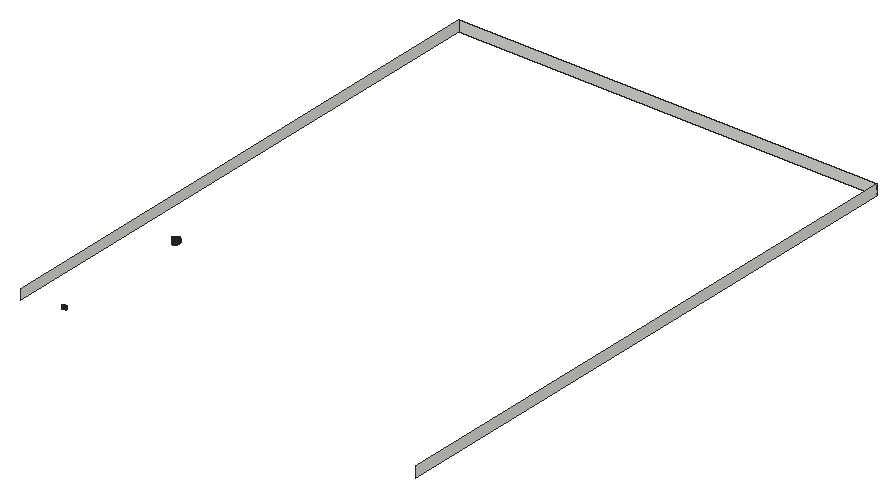
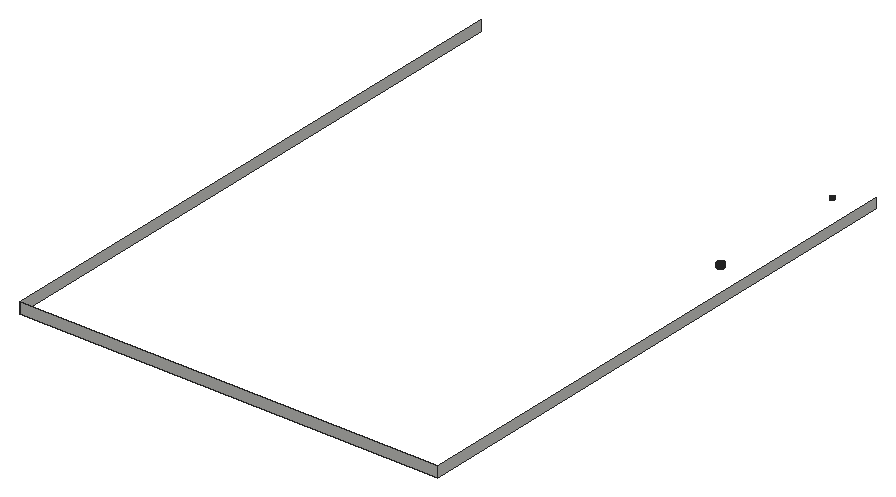
# SketchUp Ruby script. Lengths in inches.
U = 1.inch
M = Sketchup.active_model
def pt(a) = Geom::Point3d.new(a.map { |v| v * U })
def face(e, loops, mat)
  f = e.add_face(loops[0].map { |a| pt(a) })
  loops[1..].each { |l| e.add_face(l.map { |a| pt(a) }).erase! }
  f.material = f.back_material = mat if mat
  f
end
# faces: each face lists its corners as indices into pts; further lists are holes
def faces(e, pts, list, mat = nil) = list.each { |f| face(e, (f[0].is_a?(Array) ? f : [f]).map { |l| l.map { |i| pts[i] } }, mat) }
# xy, xz, yz: faces in a plane at the given z, y or x. An outline is a flat list of corners, or four numbers for a rectangle; further outlines are holes
def ring(l) = l.size == 4 ? [[l[0], l[1]], [l[2], l[1]], [l[2], l[3]], [l[0], l[3]]] : l.each_slice(2).to_a
def flat(e, list, mat, &to3) = list.each { |f| face(e, (f[0].is_a?(Array) ? f : [f]).map { |l| ring(l).map { |u, v| to3.(u, v) } }, mat) }
def xy(e, z, list, mat = nil) = flat(e, list, mat) { |x, y| [x, y, z] }
def xz(e, y, list, mat = nil) = flat(e, list, mat) { |x, z| [x, y, z] }
def yz(e, x, list, mat = nil) = flat(e, list, mat) { |y, z| [x, y, z] }
def lines(e, pts, list) = list.each { |a, b| e.add_line(pt(pts[a]), pt(pts[b])) }
# prism: a flat outline (further loops are holes) pulled along v
def prism(e, loops, v, mat = nil)
  f = face(e, loops, mat); d = Geom::Vector3d.new(v.map { |x| x * U })
  f.pushpull(f.normal.samedirection?(d) ? d.length : -d.length)
end
def box(e, o, s, mat = nil) = prism(e, [[o, [o[0] + s[0], o[1], o[2]], [o[0] + s[0], o[1] + s[1], o[2]], [o[0], o[1] + s[1], o[2]]]], [0, 0, s[2]], mat)
def at(x, y, z, deg = 0) = Geom::Transformation.translation(pt([x, y, z])) * Geom::Transformation.rotation(ORIGIN, Z_AXIS, deg.degrees)
def axes(o, x, y, z) = Geom::Transformation.new([*x, 0, *y, 0, *z, 0, *pt(o).to_a, 1])
def part(name) = M.definitions.add(name)
# library, detail: a bought-in or finely detailed component or shape, given as its bounding box
def library(name, o, s) = part(name).tap { |d| box(d.entities, o, s) }
def detail(e, o, s) = box(e.add_group.entities, o, s)
def put(e, d, t, mat = nil) = e.add_instance(d, t).tap { |i| i.material = mat if mat }
def group(e, t, mat = nil) = e.add_group.tap { |g| g.transformation = t; g.material = mat if mat }.entities
root = M.entities
M.materials.add("1122 AP 7994 PEACH ROSE").color = [254, 227, 201]
xz(root,186.05,[[40.625,149.82,40.7,152.82],[41.33,149.82,41.41,152.82]],"1122 AP 7994 PEACH ROSE")
xz(root,186.07,[[40.86,149.82,40.9375,152.82],[40.9375,149.82,41.02,152.82],[41.02,149.82,41.09,152.82],[41.09,149.82,41.17,152.82]],"1122 AP 7994 PEACH ROSE")
xz(root,300.07,[[40.86,149.82,40.9375,152.82],[40.9375,149.82,41.02,152.82],[41.02,149.82,41.09,152.82],[41.09,149.82,41.17,152.82]],"1122 AP 7994 PEACH ROSE")
xz(root,306.05,[[40.625,149.82,40.7,152.82],[41.33,149.82,41.41,152.82]],"1122 AP 7994 PEACH ROSE")
xz(root,306.07,[[40.86,149.82,40.9375,152.82],[40.9375,149.82,41.02,152.82],[41.02,149.82,41.09,152.82],[41.09,149.82,41.17,152.82]],"1122 AP 7994 PEACH ROSE")
xz(root,645,[[9,149.82,366,158.82]])
yz(root,9,[[177,149.82,645,158.82]])
yz(root,38.02,[[302.91,149.82,302.99,152.82],[302.99,149.82,303.07,152.82],[303.07,149.82,303.15,152.82],[303.15,149.82,303.23,152.82]],"1122 AP 7994 PEACH ROSE")
yz(root,38.03,[[302.76,149.82,302.84,152.82],[303.31,149.82,303.38,152.82]],"1122 AP 7994 PEACH ROSE")
yz(root,44.01,[[302.84,149.82,302.91,152.82],[303.23,149.82,303.31,152.82]],"1122 AP 7994 PEACH ROSE")
yz(root,44.02,[[302.99,149.82,303.07,152.82],[303.07,149.82,303.15,152.82]],"1122 AP 7994 PEACH ROSE")
yz(root,366,[[153,149.82,645,158.82]])
p = [[38.38,184.5,149.82],[38.42,184.57,149.82],[38.42,184.57,152.82],[38.38,184.5,152.82],[38.46,184.64,149.82],[38.46,184.64,152.82],
  [38.5,184.7,149.82],[38.5,184.7,152.82],[38.54,184.77,149.82],[38.54,184.77,152.82],[38.59,184.83,149.82],[38.59,184.83,152.82],
  [38.64,184.9,149.82],[38.64,184.9,152.82],[38.68,184.96,149.82],[38.68,184.96,152.82],[38.74,185.02,149.82],[38.74,185.02,152.82],
  [38.79,185.08,149.82],[38.79,185.08,152.82],[38.84,185.14,149.82],[38.84,185.14,152.82],[38.89,185.19,149.82],[38.89,185.19,152.82],
  [38.95,185.25,149.82],[38.95,185.25,152.82],[39.01,185.3,149.82],[39.01,185.3,152.82],[39.07,185.35,149.82],[39.07,185.35,152.82],
  [39.13,185.4,149.82],[39.13,185.4,152.82],[39.19,185.45,149.82],[39.19,185.45,152.82],[39.25,185.5,149.82],[39.25,185.5,152.82],
  [39.32,185.54,149.82],[39.32,185.54,152.82],[39.38,185.59,149.82],[39.38,185.59,152.82],[39.45,185.63,149.82],[39.45,185.63,152.82],
  [39.52,185.67,149.82],[39.52,185.67,152.82],[39.58,185.71,149.82],[39.58,185.71,152.82],[39.65,185.74,149.82],[39.65,185.74,152.82],
  [39.72,185.78,149.82],[39.72,185.78,152.82],[39.8,185.8125,149.82],[39.8,185.8125,152.82],[39.87,185.84,149.82],[39.87,185.84,152.82],
  [39.94,185.87,149.82],[39.94,185.87,152.82],[40.01,185.9,149.82],[40.01,185.9,152.82],[40.09,185.92,149.82],[40.09,185.92,152.82],
  [40.16,185.95,149.82],[40.16,185.95,152.82],[40.24,185.97,149.82],[40.24,185.97,152.82],[40.32,185.99,149.82],[40.32,185.99,152.82],
  [40.39,186.01,149.82],[40.39,186.01,152.82],[40.47,186.02,149.82],[40.47,186.02,152.82],[40.55,186.03,149.82],[40.55,186.03,152.82],
  [40.625,186.05,149.82],[40.625,186.05,152.82],[41.41,186.05,149.82],[41.49,186.03,149.82],[41.49,186.03,152.82],[41.41,186.05,152.82],
  [41.5625,186.02,149.82],[41.5625,186.02,152.82],[41.64,186.01,149.82],[41.64,186.01,152.82],[40.7,186.05,149.82],[40.78,186.0625,149.82],
  [40.78,186.0625,152.82],[40.7,186.05,152.82],[40.86,186.07,149.82],[40.86,186.07,152.82],[41.17,186.07,149.82],[41.25,186.0625,149.82],
  [41.25,186.0625,152.82],[41.17,186.07,152.82],[41.33,186.05,149.82],[41.33,186.05,152.82],[40.39,300.14,149.82],[40.32,300.15,149.82],
  [40.32,300.15,152.82],[40.39,300.14,152.82],[40.47,300.12,149.82],[40.47,300.12,152.82],[40.625,300.1,149.82],[40.55,300.11,149.82],
  [40.55,300.11,152.82],[40.625,300.1,152.82],[40.7,300.09,149.82],[40.7,300.09,152.82],[40.78,300.08,149.82],[40.78,300.08,152.82],
  [40.86,300.07,149.82],[40.86,300.07,152.82],[41.25,300.08,149.82],[41.17,300.07,149.82],[41.17,300.07,152.82],[41.25,300.08,152.82],
  [41.33,300.09,149.82],[41.33,300.09,152.82],[41.41,300.1,149.82],[41.41,300.1,152.82],[41.49,300.11,149.82],[41.49,300.11,152.82],
  [41.5625,300.12,149.82],[41.5625,300.12,152.82],[41.64,300.14,149.82],[41.64,300.14,152.82],[41.72,300.15,149.82],[41.72,300.15,152.82],
  [40.01,300.24,149.82],[39.94,300.27,149.82],[39.94,300.27,152.82],[40.01,300.24,152.82],[40.09,300.22,149.82],[40.09,300.22,152.82],
  [40.16,300.19,149.82],[40.16,300.19,152.82],[40.24,300.17,149.82],[40.24,300.17,152.82],[41.79,300.17,149.82],[41.79,300.17,152.82],
  [41.87,300.19,149.82],[41.87,300.19,152.82],[41.94,300.22,149.82],[41.94,300.22,152.82],[42.02,300.24,149.82],[42.02,300.24,152.82],
  [42.09,300.27,149.82],[42.09,300.27,152.82],[39.8,300.33,149.82],[39.72,300.36,149.82],[39.72,300.36,152.82],[39.8,300.33,152.82],
  [39.87,300.3,149.82],[39.87,300.3,152.82],[42.16,300.3,149.82],[42.16,300.3,152.82],[42.24,300.33,149.82],[42.24,300.33,152.82],
  [42.31,300.36,149.82],[42.31,300.36,152.82],[39.58,300.43,149.82],[39.52,300.47,149.82],[39.52,300.47,152.82],[39.58,300.43,152.82],
  [39.65,300.4,149.82],[39.65,300.4,152.82],[42.38,300.4,149.82],[42.38,300.4,152.82],[42.45,300.43,149.82],[42.45,300.43,152.82],
  [42.52,300.47,149.82],[42.52,300.47,152.82],[39.45,300.51,149.82],[39.45,300.51,152.82],[39.38,300.55,149.82],[39.38,300.55,152.82],
  [42.58,300.51,149.82],[42.58,300.51,152.82],[42.65,300.55,149.82],[42.65,300.55,152.82],[39.25,300.64,149.82],[39.19,300.69,149.82],
  [39.19,300.69,152.82],[39.25,300.64,152.82],[39.32,300.6,149.82],[39.32,300.6,152.82],[42.72,300.6,149.82],[42.72,300.6,152.82],
  [42.78,300.64,149.82],[42.78,300.64,152.82],[42.84,300.69,149.82],[42.84,300.69,152.82],[39.13,300.74,149.82],[39.13,300.74,152.82],
  [39.07,300.79,149.82],[39.07,300.79,152.82],[42.9,300.74,149.82],[42.9,300.74,152.82],[42.96,300.79,149.82],[42.96,300.79,152.82],
  [39.01,300.84,149.82],[39.01,300.84,152.82],[38.95,300.89,149.82],[38.95,300.89,152.82],[43.02,300.84,149.82],[43.02,300.84,152.82],
  [43.08,300.89,149.82],[43.08,300.89,152.82],[38.89,300.95,149.82],[38.84,301.01,149.82],[38.84,301.01,152.82],[38.89,300.95,152.82],
  [43.14,300.95,149.82],[43.14,300.95,152.82],[43.19,301.01,149.82],[43.19,301.01,152.82],[38.79,301.0625,149.82],[38.79,301.0625,152.82],
  [43.25,301.0625,149.82],[43.25,301.0625,152.82],[38.74,301.12,149.82],[38.74,301.12,152.82],[38.68,301.18,149.82],[38.68,301.18,152.82],
  [43.3,301.12,149.82],[43.3,301.12,152.82],[43.35,301.18,149.82],[43.35,301.18,152.82],[38.64,301.24,149.82],[38.64,301.24,152.82],
  [38.59,301.31,149.82],[38.59,301.31,152.82],[43.4,301.24,149.82],[43.4,301.24,152.82],[43.44,301.31,149.82],[43.44,301.31,152.82],
  [38.54,301.37,149.82],[38.54,301.37,152.82],[43.49,301.37,149.82],[43.49,301.37,152.82],[38.5,301.4375,149.82],[38.5,301.4375,152.82],
  [38.46,301.5,149.82],[38.46,301.5,152.82],[43.53,301.4375,149.82],[43.53,301.4375,152.82],[43.57,301.5,149.82],[43.57,301.5,152.82],
  [38.42,301.57,149.82],[38.42,301.57,152.82],[43.61,301.57,149.82],[43.61,301.57,152.82],[38.38,301.64,149.82],[38.34,301.71,149.82],
  [38.34,301.71,152.82],[38.38,301.64,152.82],[43.65,301.64,149.82],[43.65,301.64,152.82],[43.6875,301.71,149.82],[43.6875,301.71,152.82],
  [38.31,301.78,149.82],[38.31,301.78,152.82],[43.72,301.78,149.82],[43.72,301.78,152.82],[38.28,301.85,149.82],[38.28,301.85,152.82],
  [43.76,301.85,149.82],[43.76,301.85,152.82],[38.24,301.92,149.82],[38.24,301.92,152.82],[38.22,302,149.82],[38.22,302,152.82],
  [43.79,301.92,149.82],[43.79,301.92,152.82],[43.82,302,149.82],[43.82,302,152.82],[38.1875,302.07,149.82],[38.1875,302.07,152.82],
  [43.84,302.07,149.82],[43.84,302.07,152.82],[38.16,302.14,149.82],[38.14,302.22,149.82],[38.14,302.22,152.82],[38.16,302.14,152.82],
  [43.87,302.14,149.82],[43.87,302.14,152.82],[43.89,302.22,149.82],[43.89,302.22,152.82],[38.12,302.29,149.82],[38.12,302.29,152.82],
  [43.91,302.29,149.82],[43.91,302.29,152.82],[38.1,302.37,149.82],[38.1,302.37,152.82],[43.93,302.37,149.82],[43.93,302.37,152.82],
  [38.08,302.45,149.82],[38.08,302.45,152.82],[38.07,302.52,149.82],[38.07,302.52,152.82],[43.95,302.45,149.82],[43.95,302.45,152.82],
  [43.97,302.52,149.82],[43.97,302.52,152.82],[38.05,302.6,149.82],[38.05,302.6,152.82],[43.98,302.6,149.82],[43.98,302.6,152.82],
  [38.04,302.68,149.82],[38.04,302.68,152.82],[43.99,302.68,149.82],[43.99,302.68,152.82],[38.03,302.76,149.82],[38.03,302.76,152.82],
  [44,302.76,149.82],[44,302.76,152.82],[38.03,302.84,149.82],[38.02,302.91,149.82],[38.02,302.91,152.82],[38.03,302.84,152.82],
  [44.01,302.84,149.82],[44.01,302.84,152.82],[44.02,302.99,149.82],[44.01,302.91,149.82],[44.01,302.91,152.82],[44.02,302.99,152.82],
  [44.01,303.23,149.82],[44.02,303.15,149.82],[44.02,303.15,152.82],[44.01,303.23,152.82],[38.02,303.23,149.82],[38.03,303.31,149.82],
  [38.03,303.31,152.82],[38.02,303.23,152.82],[44,303.38,149.82],[44.01,303.31,149.82],[44.01,303.31,152.82],[44,303.38,152.82],
  [38.03,303.38,149.82],[38.04,303.46,149.82],[38.04,303.46,152.82],[38.03,303.38,152.82],[43.99,303.46,149.82],[43.99,303.46,152.82],
  [38.05,303.54,149.82],[38.05,303.54,152.82],[38.07,303.62,149.82],[38.07,303.62,152.82],[43.98,303.54,149.82],[43.98,303.54,152.82],
  [43.97,303.62,149.82],[43.97,303.62,152.82],[38.08,303.69,149.82],[38.08,303.69,152.82],[43.95,303.69,149.82],[43.95,303.69,152.82],
  [38.1,303.77,149.82],[38.1,303.77,152.82],[43.93,303.77,149.82],[43.93,303.77,152.82],[38.12,303.85,149.82],[38.12,303.85,152.82],
  [38.14,303.92,149.82],[38.14,303.92,152.82],[43.91,303.85,149.82],[43.91,303.85,152.82],[43.89,303.92,149.82],[43.89,303.92,152.82],
  [38.16,304,149.82],[38.16,304,152.82],[43.87,304,149.82],[43.87,304,152.82],[38.1875,304.07,149.82],[38.1875,304.07,152.82],
  [43.84,304.07,149.82],[43.84,304.07,152.82],[38.22,304.15,149.82],[38.22,304.15,152.82],[38.24,304.22,149.82],[38.24,304.22,152.82],
  [43.82,304.15,149.82],[43.82,304.15,152.82],[43.79,304.22,149.82],[43.79,304.22,152.82],[38.28,304.29,149.82],[38.28,304.29,152.82],
  [43.76,304.29,149.82],[43.76,304.29,152.82],[38.31,304.36,149.82],[38.31,304.36,152.82],[43.72,304.36,149.82],[43.72,304.36,152.82],
  [38.34,304.43,149.82],[38.34,304.43,152.82],[38.38,304.5,149.82],[38.38,304.5,152.82],[43.6875,304.43,149.82],[43.6875,304.43,152.82],
  [43.65,304.5,149.82],[43.65,304.5,152.82],[38.42,304.57,149.82],[38.42,304.57,152.82],[43.61,304.57,149.82],[43.61,304.57,152.82],
  [38.46,304.64,149.82],[38.46,304.64,152.82],[38.5,304.7,149.82],[38.5,304.7,152.82],[43.53,304.7,149.82],[43.57,304.64,149.82],
  [43.57,304.64,152.82],[43.53,304.7,152.82],[38.54,304.77,149.82],[38.54,304.77,152.82],[43.49,304.77,149.82],[43.49,304.77,152.82],
  [38.59,304.83,149.82],[38.59,304.83,152.82],[38.64,304.9,149.82],[38.64,304.9,152.82],[43.44,304.83,149.82],[43.44,304.83,152.82],
  [43.4,304.9,149.82],[43.4,304.9,152.82],[38.68,304.96,149.82],[38.68,304.96,152.82],[43.35,304.96,149.82],[43.35,304.96,152.82],
  [38.74,305.02,149.82],[38.74,305.02,152.82],[38.79,305.08,149.82],[38.79,305.08,152.82],[43.25,305.08,149.82],[43.3,305.02,149.82],
  [43.3,305.02,152.82],[43.25,305.08,152.82],[38.84,305.14,149.82],[38.84,305.14,152.82],[38.89,305.19,149.82],[38.89,305.19,152.82],
  [43.14,305.19,149.82],[43.19,305.14,149.82],[43.19,305.14,152.82],[43.14,305.19,152.82],[38.95,305.25,149.82],[38.95,305.25,152.82],
  [39.01,305.3,149.82],[39.01,305.3,152.82],[43.02,305.3,149.82],[43.08,305.25,149.82],[43.08,305.25,152.82],[43.02,305.3,152.82],
  [39.07,305.35,149.82],[39.07,305.35,152.82],[42.96,305.35,149.82],[42.96,305.35,152.82],[39.13,305.4,149.82],[39.13,305.4,152.82],
  [39.19,305.45,149.82],[39.19,305.45,152.82],[42.84,305.45,149.82],[42.9,305.4,149.82],[42.9,305.4,152.82],[42.84,305.45,152.82],
  [39.25,305.5,149.82],[39.25,305.5,152.82],[39.32,305.54,149.82],[39.32,305.54,152.82],[39.38,305.59,149.82],[39.38,305.59,152.82],
  [42.72,305.54,149.82],[42.78,305.5,149.82],[42.78,305.5,152.82],[42.72,305.54,152.82],[42.65,305.59,149.82],[42.65,305.59,152.82],
  [39.45,305.63,149.82],[39.45,305.63,152.82],[39.52,305.67,149.82],[39.52,305.67,152.82],[42.52,305.67,149.82],[42.58,305.63,149.82],
  [42.58,305.63,152.82],[42.52,305.67,152.82],[39.58,305.71,149.82],[39.58,305.71,152.82],[39.65,305.74,149.82],[39.65,305.74,152.82],
  [39.72,305.78,149.82],[39.72,305.78,152.82],[42.31,305.78,149.82],[42.38,305.74,149.82],[42.38,305.74,152.82],[42.31,305.78,152.82],
  [42.45,305.71,149.82],[42.45,305.71,152.82],[39.8,305.8125,149.82],[39.8,305.8125,152.82],[39.87,305.84,149.82],[39.87,305.84,152.82],
  [39.94,305.87,149.82],[39.94,305.87,152.82],[42.09,305.87,149.82],[42.16,305.84,149.82],[42.16,305.84,152.82],[42.09,305.87,152.82],
  [42.24,305.8125,149.82],[42.24,305.8125,152.82],[40.01,305.9,149.82],[40.01,305.9,152.82],[40.09,305.92,149.82],[40.09,305.92,152.82],
  [40.16,305.95,149.82],[40.16,305.95,152.82],[40.24,305.97,149.82],[40.24,305.97,152.82],[41.79,305.97,149.82],[41.87,305.95,149.82],
  [41.87,305.95,152.82],[41.79,305.97,152.82],[41.94,305.92,149.82],[42.02,305.9,149.82],[42.02,305.9,152.82],[41.94,305.92,152.82],
  [40.32,305.99,149.82],[40.32,305.99,152.82],[40.39,306.01,149.82],[40.39,306.01,152.82],[40.47,306.02,149.82],[40.47,306.02,152.82],
  [40.55,306.03,149.82],[40.55,306.03,152.82],[40.625,306.05,149.82],[40.625,306.05,152.82],[41.41,306.05,149.82],[41.49,306.03,149.82],
  [41.49,306.03,152.82],[41.41,306.05,152.82],[41.5625,306.02,149.82],[41.5625,306.02,152.82],[41.64,306.01,149.82],[41.72,305.99,149.82],
  [41.72,305.99,152.82],[41.64,306.01,152.82],[40.7,306.05,149.82],[40.78,306.0625,149.82],[40.78,306.0625,152.82],[40.7,306.05,152.82],
  [40.86,306.07,149.82],[40.86,306.07,152.82],[41.17,306.07,149.82],[41.25,306.0625,149.82],[41.25,306.0625,152.82],[41.17,306.07,152.82],
  [41.33,306.05,149.82],[41.33,306.05,152.82]]
faces(root,p,[[0,1,2,3],[1,4,5,2],[4,6,7,5],[6,8,9,7],[8,10,11,9],[10,12,13,11],[12,14,15,13],[14,16,17,15],
  [16,18,19,17],[18,20,21,19],[20,22,23,21],[22,24,25,23],[24,26,27,25],[26,28,29,27],[28,30,31,29],[30,32,33,31],
  [32,34,35,33],[34,36,37,35],[36,38,39,37],[38,40,41,39],[40,42,43,41],[42,44,45,43],[44,46,47,45],[46,48,49,47],
  [48,50,51,49],[50,52,53,51],[52,54,55,53],[54,56,57,55],[56,58,59,57],[58,60,61,59],[60,62,63,61],[62,64,65,63],
  [64,66,67,65],[66,68,69,67],[68,70,71,69],[70,72,73,71],[74,75,76,77],[75,78,79,76],[78,80,81,79],[82,83,84,85],
  [83,86,87,84],[88,89,90,91],[89,92,93,90],[94,95,96,97],[98,94,97,99],[100,101,102,103],[101,98,99,102],[104,100,103,105],
  [106,104,105,107],[108,106,107,109],[110,111,112,113],[114,110,113,115],[116,114,115,117],[118,116,117,119],[120,118,119,121],[122,120,121,123],
  [124,122,123,125],[126,127,128,129],[130,126,129,131],[132,130,131,133],[95,134,135,96],[134,132,133,135],[136,124,125,137],[138,136,137,139],
  [140,138,139,141],[142,140,141,143],[144,142,143,145],[146,147,148,149],[150,146,149,151],[127,150,151,128],[152,144,145,153],[154,152,153,155],
  [156,154,155,157],[158,159,160,161],[162,158,161,163],[147,162,163,148],[164,156,157,165],[166,164,165,167],[168,166,167,169],[159,170,171,160],
  [170,172,173,171],[174,168,169,175],[176,174,175,177],[178,179,180,181],[172,182,183,173],[182,178,181,183],[184,176,177,185],[186,184,185,187],
  [188,186,187,189],[179,190,191,180],[190,192,193,191],[194,188,189,195],[196,194,195,197],[192,198,199,193],[198,200,201,199],[202,196,197,203],
  [204,202,203,205],[206,207,208,209],[200,206,209,201],[210,204,205,211],[212,210,211,213],[207,214,215,208],[216,212,213,217],[214,218,219,215],
  [218,220,221,219],[222,216,217,223],[224,222,223,225],[220,226,227,221],[226,228,229,227],[230,224,225,231],[232,230,231,233],[228,234,235,229],
  [236,232,233,237],[234,238,239,235],[238,240,241,239],[242,236,237,243],[244,242,243,245],[240,246,247,241],[248,244,245,249],[250,251,252,253],
  [246,250,253,247],[254,248,249,255],[256,254,255,257],[251,258,259,252],[260,256,257,261],[258,262,263,259],[264,260,261,265],[262,266,267,263],
  [266,268,269,267],[270,264,265,271],[272,270,271,273],[268,274,275,269],[276,272,273,277],[278,279,280,281],[274,278,281,275],[282,276,277,283],
  [284,282,283,285],[279,286,287,280],[288,284,285,289],[286,290,291,287],[292,288,289,293],[290,294,295,291],[294,296,297,295],[298,292,293,299],
  [300,298,299,301],[296,302,303,297],[304,300,301,305],[302,306,307,303],[308,304,305,309],[306,310,311,307],[312,308,309,313],[314,315,316,317],
  [318,312,313,319],[320,321,322,323],[324,325,326,327],[328,329,330,331],[332,333,334,335],[336,337,338,339],[340,332,335,341],[337,342,343,338],
  [342,344,345,343],[346,340,341,347],[348,346,347,349],[344,350,351,345],[352,348,349,353],[350,354,355,351],[356,352,353,357],[354,358,359,355],
  [358,360,361,359],[362,356,357,363],[364,362,363,365],[360,366,367,361],[368,364,365,369],[366,370,371,367],[372,368,369,373],[370,374,375,371],
  [374,376,377,375],[378,372,373,379],[380,378,379,381],[376,382,383,377],[384,380,381,385],[382,386,387,383],[388,384,385,389],[386,390,391,387],
  [390,392,393,391],[394,388,389,395],[396,394,395,397],[392,398,399,393],[400,396,397,401],[398,402,403,399],[402,404,405,403],[406,407,408,409],
  [407,400,401,408],[404,410,411,405],[412,406,409,413],[410,414,415,411],[414,416,417,415],[418,412,413,419],[420,418,419,421],[416,422,423,417],
  [424,420,421,425],[422,426,427,423],[426,428,429,427],[430,431,432,433],[431,424,425,432],[428,434,435,429],[434,436,437,435],[438,439,440,441],
  [439,430,433,440],[436,442,443,437],[442,444,445,443],[446,447,448,449],[447,438,441,448],[444,450,451,445],[452,446,449,453],[450,454,455,451],
  [454,456,457,455],[458,459,460,461],[459,452,453,460],[456,462,463,457],[462,464,465,463],[464,466,467,465],[468,469,470,471],[472,468,471,473],
  [469,458,461,470],[466,474,475,467],[474,476,477,475],[478,479,480,481],[479,472,473,480],[476,482,483,477],[482,484,485,483],[484,486,487,485],
  [488,489,490,491],[492,478,481,493],[489,492,493,490],[486,494,495,487],[494,496,497,495],[496,498,499,497],[500,501,502,503],[504,488,491,505],
  [501,504,505,502],[498,506,507,499],[506,508,509,507],[508,510,511,509],[510,512,513,511],[514,515,516,517],[518,519,520,521],[515,518,521,516],
  [519,500,503,520],[512,522,523,513],[522,524,525,523],[524,526,527,525],[526,528,529,527],[528,530,531,529],[532,533,534,535],[533,536,537,534],
  [538,539,540,541],[536,538,541,537],[539,514,517,540],[542,543,544,545],[543,546,547,544],[548,549,550,551],[549,552,553,550]],"1122 AP 7994 PEACH ROSE")
